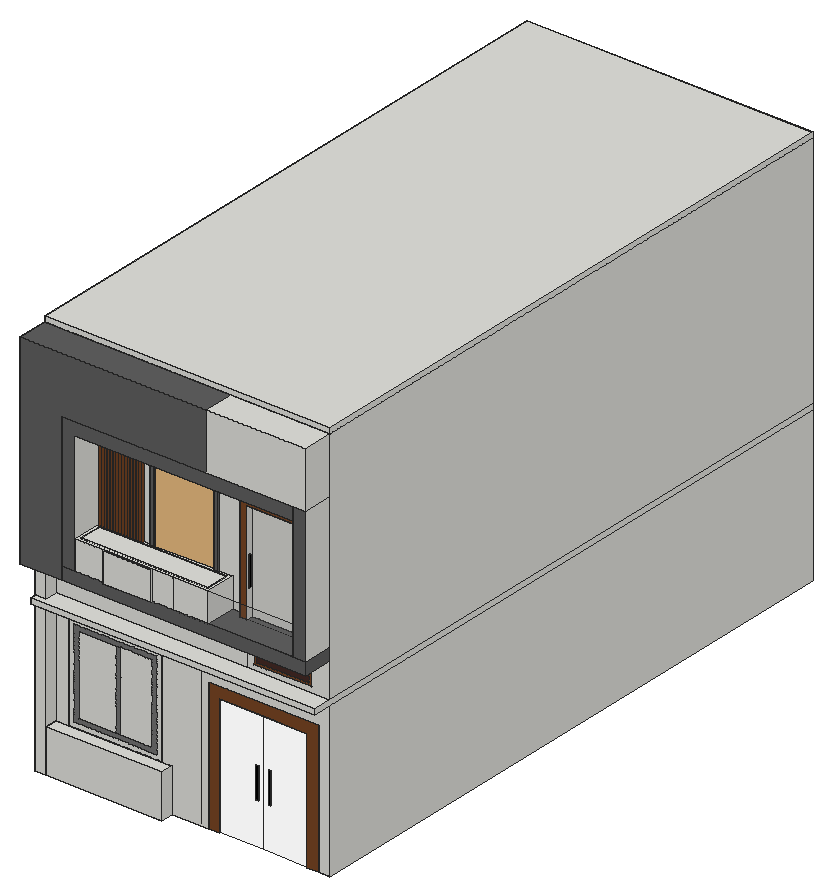
# SketchUp Ruby script. Lengths in inches.
U = 1.inch
M = Sketchup.active_model
def pt(a) = Geom::Point3d.new(a.map { |v| v * U })
def face(e, loops, mat)
  f = e.add_face(loops[0].map { |a| pt(a) })
  loops[1..].each { |l| e.add_face(l.map { |a| pt(a) }).erase! }
  f.material = f.back_material = mat if mat
  f
end
# faces: each face lists its corners as indices into pts; further lists are holes
def faces(e, pts, list, mat = nil) = list.each { |f| face(e, (f[0].is_a?(Array) ? f : [f]).map { |l| l.map { |i| pts[i] } }, mat) }
# xy, xz, yz: faces in a plane at the given z, y or x. An outline is a flat list of corners, or four numbers for a rectangle; further outlines are holes
def ring(l) = l.size == 4 ? [[l[0], l[1]], [l[2], l[1]], [l[2], l[3]], [l[0], l[3]]] : l.each_slice(2).to_a
def flat(e, list, mat, &to3) = list.each { |f| face(e, (f[0].is_a?(Array) ? f : [f]).map { |l| ring(l).map { |u, v| to3.(u, v) } }, mat) }
def xy(e, z, list, mat = nil) = flat(e, list, mat) { |x, y| [x, y, z] }
def xz(e, y, list, mat = nil) = flat(e, list, mat) { |x, z| [x, y, z] }
def yz(e, x, list, mat = nil) = flat(e, list, mat) { |y, z| [x, y, z] }
def lines(e, pts, list) = list.each { |a, b| e.add_line(pt(pts[a]), pt(pts[b])) }
# prism: a flat outline (further loops are holes) pulled along v
def prism(e, loops, v, mat = nil)
  f = face(e, loops, mat); d = Geom::Vector3d.new(v.map { |x| x * U })
  f.pushpull(f.normal.samedirection?(d) ? d.length : -d.length)
end
def box(e, o, s, mat = nil) = prism(e, [[o, [o[0] + s[0], o[1], o[2]], [o[0] + s[0], o[1] + s[1], o[2]], [o[0], o[1] + s[1], o[2]]]], [0, 0, s[2]], mat)
def at(x, y, z, deg = 0) = Geom::Transformation.translation(pt([x, y, z])) * Geom::Transformation.rotation(ORIGIN, Z_AXIS, deg.degrees)
def axes(o, x, y, z) = Geom::Transformation.new([*x, 0, *y, 0, *z, 0, *pt(o).to_a, 1])
def part(name) = M.definitions.add(name)
# library, detail: a bought-in or finely detailed component or shape, given as its bounding box
def library(name, o, s) = part(name).tap { |d| box(d.entities, o, s) }
def detail(e, o, s) = box(e.add_group.entities, o, s)
def put(e, d, t, mat = nil) = e.add_instance(d, t).tap { |i| i.material = mat if mat }
def group(e, t, mat = nil) = e.add_group.tap { |g| g.transformation = t; g.material = mat if mat }.entities
root = M.entities
M.materials.add("Lily_Dark").color = [68, 42, 38]
M.materials.add("Material12").color = [68, 110, 58]
M.materials.add("Material13").color = [48, 90, 38]
M.materials.add("Material14").color = [68, 110, 48]
M.materials.add("Material15").color = [48, 90, 48]
M.materials.add("Material16").color = [58, 110, 58]
M.materials.add("Material17").color = [58, 90, 38]
M.materials.add("Material18").color = [68, 100, 58]
M.materials.add("Material19").color = [48, 100, 38]
M.materials.add("Material~1").color = [96, 96, 96]
M.materials.add("[Color M05]").color = [114, 114, 114]
M.materials.add("[Color M09]").color = [0, 0, 0]
M.materials.add("[Color_000]").color = [255, 255, 255]
M.materials.add("[Color_009]").color = [0, 0, 0]
M.materials.add("[Groundcover_BarkChips]").color = [119, 116, 116]
M.materials.add("[Translucent Glass Gray]").color = [128, 128, 128]
M.materials["[Translucent Glass Gray]"].alpha = 0.1
M.materials.add("[Wood Veneer 01]").color = [120, 70, 37]
M.materials.add("stainless-steel").color = [0, 0, 0]
c1 = part("Corrugated panel")
box(c1.entities,[0,-2,0],[0.29,2,87.84])
box(c1.entities,[2.25,-2,0],[0.29,2,87.84])
box(c1.entities,[4.5,-2,0],[0.29,2,87.84])
box(c1.entities,[6.75,-2,0],[0.29,2,87.84])
box(c1.entities,[9,-2,0],[0.29,2,87.84])
box(c1.entities,[11.25,-2,0],[0.29,2,87.84])
box(c1.entities,[13.5,-2,0],[0.29,2,87.84])
box(c1.entities,[15.75,-2,0],[0.29,2,87.84])
box(c1.entities,[18,-2,0],[0.29,2,87.84])
box(c1.entities,[20.25,-2,0],[0.29,2,87.84])
box(c1.entities,[22.5,-2,0],[0.29,2,87.84])
box(c1.entities,[24.75,-2,0],[0.29,2,87.84])
box(c1.entities,[27,-2,0],[0.29,2,87.84])
box(c1.entities,[29.25,-2,0],[0.29,2,87.84])
box(c1.entities,[31.5,-2,0],[0.29,2,87.84])
box(c1.entities,[33.75,-2,0],[0.29,2,87.84])
box(c1.entities,[36,-2,0],[0.29,2,87.84])
box(c1.entities,[38.25,-2,0],[0.29,2,87.84])
box(c1.entities,[40.5,-2,0],[0.29,2,87.84])
box(c1.entities,[42.75,-2,0],[0.29,2,87.84])
box(c1.entities,[45,-2,0],[0.29,2,87.84])
c2 = library("Entrance door assembly",[-0.84,0,0],[9.1,39.62,78.08])
c3 = part("grass00")
p = [[-0.6875,0.15,0],[-0.56,0.08,5.52],[-0.04,0.03,2.76],[0.48,-0.02,0],[0.35,-0.02,5.52],[-0.1,-0.14,5.52],
  [-0.12,0.65,8.37],[-0.42,0.65,8.37]]
faces(c3.entities,p,[[0,1,2,3],[3,2,4],[1,5,2],[5,4,2],[1,6,5],[4,5,6],[7,6,1]])
c4 = part("Group108\#1")
put(c4.entities,c3,axes([-0.58,1.48,-0.01],[-0.26105,-0.10256,0],[0.0935,-0.23799,0.11527],[-0.04215,0.10729,0.25569]),"Material13")
put(c4.entities,c3,axes([-0.52,0.79,-0.01],[-0.30673,-0.20262,0],[0.17042,-0.25799,0.19884],[-0.1096,0.16591,0.30919]),"Material19")
put(c4.entities,c3,axes([-1.29,1.27,-0.01],[-0.1009,-0.10249,0],[0.10193,-0.10034,0.01514],[-0.01079,0.01062,0.14303]),"Material12")
put(c4.entities,c3,axes([-1.58,1.01,-0.01],[-0.09481,-0.14853,0],[0.12966,-0.08276,0.08597],[-0.07246,0.04626,0.15382]))
put(c4.entities,c3,axes([-0.85,0.32,-0.01],[-0.07211,-0.19233,0],[0.17265,-0.06473,0.09052],[-0.08476,0.03178,0.18439]),"Material16")
put(c4.entities,c3,axes([-1.06,0.16,-0.01],[-0.03023,-0.20103,0],[0.19643,-0.02954,0.04326],[-0.04278,0.00643,0.19863]),"Material17")
put(c4.entities,c3,axes([-1.78,-0.11,-0.01],[0.01133,-0.18805,0],[0.18159,0.01094,0.04894],[-0.04885,-0.00294,0.18192]),"Material19")
put(c4.entities,c3,axes([-1.57,-0.43,-0.01],[0.06705,-0.24264,0],[0.22711,0.06276,0.08862],[-0.08542,-0.02361,0.23562]),"Material14")
put(c4.entities,c3,axes([-0.97,-0.51,-0.01],[0.07163,-0.1379,0],[0.1379,0.07163,0.00033],[-0.00029,-0.00015,0.15539]),"Material16")
put(c4.entities,c3,axes([-0.55,-0.45,-0.01],[0.22039,-0.26784,0],[0.17095,0.14066,0.26702],[-0.20619,-0.16966,0.22138]),"Material19")
put(c4.entities,c3,axes([-0.66,-0.83,-0.01],[0.15006,-0.11959,0],[0.10592,0.13291,0.08908],[-0.05552,-0.06966,0.16995]),"Material19")
put(c4.entities,c3,axes([-0.36,-0.72,-0.01],[0.33439,-0.1671,0],[0.1176,0.23533,0.26558],[-0.11871,-0.23757,0.26308]),"Material12")
put(c4.entities,c3,axes([-0.17,-0.64,-0.01],[0.32333,-0.08393,0],[0.04214,0.16232,0.2889],[-0.07259,-0.27963,0.1677]))
put(c4.entities,c3,axes([-0.04,-0.9,-0.01],[0.26603,-0.01186,0],[0.01186,0.26603,0.00131],[-0.00006,-0.00131,0.26629]),"Material16")
put(c4.entities,c3,axes([0.21,-1.24,-0.01],[0.19373,0.03224,0],[-0.02742,0.16477,0.10329],[0.01696,-0.10189,0.16703]))
put(c4.entities,c3,axes([0.58,-1.47,-0.01],[0.27421,0.10773,0],[-0.06718,0.171,0.23031],[0.08421,-0.21436,0.18372]),"Material17")
put(c4.entities,c3,axes([1.01,-1.53,-0.01],[0.182,0.12023,0],[-0.11708,0.17724,0.04956],[0.02732,-0.04135,0.21242]),"Material15")
put(c4.entities,c3,axes([1.13,-1.11,-0.01],[0.08993,0.09135,0],[-0.04886,0.0481,0.10832],[0.07719,-0.07599,0.06856]),"Material16")
put(c4.entities,c3,axes([0.57,-0.37,-0.01],[0.13107,0.20532,0],[-0.17134,0.10937,0.13423],[0.11314,-0.07222,0.20327]),"Material14")
put(c4.entities,c3,axes([1.17,-0.44,-0.01],[0.12226,0.32609,0],[-0.18227,0.06833,0.28877],[0.27039,-0.10137,0.19466]),"Material12")
put(c4.entities,c3,axes([0.79,-0.12,-0.01],[0.04726,0.31426,0],[-0.23697,0.03563,0.20873],[0.20641,-0.03104,0.23963]),"Material13")
put(c4.entities,c3,axes([1.11,0.07,-0.01],[-0.00983,0.16317,0],[-0.12959,-0.00781,0.09932],[0.09914,0.00597,0.12983]),"Material15")
put(c4.entities,c3,axes([1.34,0.37,-0.01],[-0.077,0.27862,0],[-0.26284,-0.07264,0.09592],[0.09245,0.02555,0.27269]),"Material18")
put(c4.entities,c3,axes([1.43,0.74,-0.01],[-0.09818,0.18902,0],[-0.17019,-0.0884,0.09267],[0.08224,0.04272,0.19178]),"Material15")
put(c4.entities,c3,axes([0.68,0.56,-0.01],[-0.19396,0.23573,0],[-0.19529,-0.16069,0.17096],[0.13201,0.10862,0.2529]),"Material17")
put(c4.entities,c3,axes([1.13,1.42,-0.01],[-0.175,0.13946,0],[-0.12896,-0.16183,0.08516],[0.05308,0.0666,0.20693]),"Material19")
put(c4.entities,c3,axes([0.57,1.15,-0.01],[-0.14357,0.07174,0],[-0.03981,-0.07966,0.13353],[0.05969,0.11944,0.08905]),"Material19")
put(c4.entities,c3,axes([0.42,1.63,-0.01],[-0.19191,0.04982,0],[-0.03576,-0.13775,0.13805],[0.03469,0.13362,0.14232]))
put(c4.entities,c3,axes([0.05,1.02,-0.01],[-0.23102,0.0103,0],[-0.00712,-0.15969,0.1671],[0.00744,0.16694,0.15985]),"Material12")
put(c4.entities,c3,axes([-0.24,1.45,-0.01],[-0.18944,-0.03152,0],[0.03127,-0.1879,0.02439],[-0.004,0.02405,0.19049]),"Material15")
c5 = part("Group107\#1")
put(c5.entities,c4,at(0,0,0))
c6 = part("3darcstudiotree_grass00")
put(c6.entities,c5,at(0,0,0))
c7 = part("Group104\#1")
put(c7.entities,c6,axes([121.2,-0.39,1.37],[-1.04345,0.21132,0],[-0.2343,-1.15691,-0.03532],[-0.00931,-0.04597,1.5674]))
put(c7.entities,c6,axes([126.74,-0.5,1.37],[-0.81222,-0.535,0],[0.66881,-1.01537,-0.05333],[0.03791,-0.05756,1.57138]))
put(c7.entities,c6,axes([116.24,-0.29,1.37],[0.45586,-0.8369,0],[1.087,0.59209,-0.05145],[0.05418,0.02951,1.48449]))
put(c7.entities,c6,axes([129.92,-1.13,1.37],[0.5987,0.96121,0],[-0.80897,0.50387,-0.01309],[-0.01852,0.01154,1.58919]))
put(c7.entities,c6,axes([112.39,-0.41,1.37],[-0.41741,-1.14553,0],[0.92662,-0.33764,-0.04573],[0.06587,-0.024,1.51206]))
put(c7.entities,c6,axes([132.01,-1.1,1.37],[1.1241,-0.29373,0],[0.24406,0.934,-0.01529],[0.00612,0.02342,1.52853]))
put(c7.entities,c6,axes([109.24,-1.23,1.37],[0.10575,1.00852,0],[-1.03726,0.10876,-0.00707],[-0.01059,0.00111,1.57151]))
put(c7.entities,c6,axes([123.48,-1.1875,1.37],[-1.04345,0.21132,0],[-0.2343,-1.15691,-0.03532],[-0.00931,-0.04597,1.5674]))
put(c7.entities,c6,axes([119.28,-1.1875,1.37],[-1.04345,0.21132,0],[-0.2343,-1.15691,-0.03532],[-0.00931,-0.04597,1.5674]))
put(c7.entities,c6,axes([115.03,-1.13,1.37],[0.45586,-0.8369,0],[1.087,0.59209,-0.05145],[0.05418,0.02951,1.48449]))
c8 = part("Grass planter")
xy(c8.entities,0,[[[0.37,1.03,27.93,6.94],[0.77,1.43,27.54,6.55]]],"[Color_000]")
xy(c8.entities,1.37,[[0.77,1.43,27.54,6.55]],"[Groundcover_BarkChips]")
xy(c8.entities,1.57,[[[0.37,1.03,27.93,6.94],[0.77,1.43,27.54,6.55]]],"[Color_009]")
xz(c8.entities,1.03,[[0.37,0,27.93,1.57]])
xz(c8.entities,1.43,[[0.77,0,27.54,1.37]],"[Color_000]")
xz(c8.entities,1.43,[[0.77,1.37,27.54,1.57]],"[Color_009]")
xz(c8.entities,6.55,[[0.77,0,27.54,1.37]],"[Color_000]")
xz(c8.entities,6.55,[[0.77,1.37,27.54,1.57]],"[Color_009]")
xz(c8.entities,6.94,[[0.37,0,27.93,1.57]])
yz(c8.entities,0.37,[[1.03,0,6.94,1.57]])
yz(c8.entities,0.77,[[1.43,0,6.55,1.37]],"[Color_000]")
yz(c8.entities,0.77,[[1.43,1.37,6.55,1.57]],"[Color_009]")
yz(c8.entities,27.54,[[1.43,0,6.55,1.37]],"[Color_000]")
yz(c8.entities,27.54,[[1.43,1.37,6.55,1.57]],"[Color_009]")
yz(c8.entities,27.93,[[1.03,0,6.94,1.57]])
put(c8.entities,c7,at(-106.55,4.625,0))
c9 = part("Difference\#2")
xy(c9.entities,0,[[0,0,0,473,223.84,473,223.84,0,214.84,0,214.84,464,9,464,9,9,128.52,9,128.52,0]])
xy(c9.entities,34,[[19.21,0,92.04,9]])
xy(c9.entities,103,[[128.52,0,214.84,9]])
xy(c9.entities,111,[[19.21,0,92.04,9]])
xy(c9.entities,120,[[[0,0,223.84,473],[9,9,214.84,464]]])
xz(c9.entities,0,[[[0,0,128.52,0,128.52,103,214.84,103,214.84,0,223.84,0,223.84,120,0,120],[19.21,34,92.04,111]]])
xz(c9.entities,9,[[[9,0,9,120,214.84,120,214.84,103,128.52,103,128.52,0],[19.21,34,92.04,111]]])
xz(c9.entities,464,[[9,0,214.84,120]])
xz(c9.entities,473,[[0,0,223.84,120]])
yz(c9.entities,0,[[0,0,473,120]])
yz(c9.entities,9,[[9,0,464,120]])
yz(c9.entities,19.21,[[0,34,9,111]])
yz(c9.entities,92.04,[[0,34,9,111]])
yz(c9.entities,128.52,[[0,0,9,103]])
yz(c9.entities,214.84,[[0,0,9,103],[9,0,464,120]])
yz(c9.entities,223.84,[[0,0,473,120]])
p = [[123.02,0,1.98],[123.02,0,120]]
lines(c9.entities,p,[[0,1]])
c10 = part("Difference\#1")
xy(c10.entities,0,[[0,0,0,473,223.84,473,223.84,0,128.52,0,128.52,9,214.84,9,214.84,464,9,464,9,9,128.52,9,128.52,0]])
xy(c10.entities,48.19,[[86.57,0,133.57,9]])
xy(c10.entities,122.19,[[86.57,0,133.57,9]])
xy(c10.entities,187,[[[0,0,223.84,473],[9,9,214.84,464]]])
xz(c10.entities,0,[[[0,0,158.62,0,158.62,27.47,223.84,27.47,223.84,187,0,187],[86.57,48.19,133.57,122.19]]])
xz(c10.entities,9,[[[9,0,214.84,187],[86.57,48.19,133.57,122.19]]])
xz(c10.entities,464,[[9,0,214.84,187]])
xz(c10.entities,473,[[0,0,223.84,187]])
yz(c10.entities,0,[[0,0,473,187]])
yz(c10.entities,9,[[9,0,464,187]])
yz(c10.entities,86.57,[[0,48.19,9,122.19]])
yz(c10.entities,133.57,[[0,48.19,9,122.19]])
yz(c10.entities,214.84,[[9,0,464,187]])
yz(c10.entities,223.84,[[0,0,473,187]])
p = [[124.34,0,27.47],[119.51,0,27.47],[131.53,0,27.47],[126.28,0,27.47]]
lines(c10.entities,p,[[0,1],[2,3]])
g1 = group(c10.entities,at(158.62,0,0))
xz(g1,0,[[[0,0,65.22,27.47],[5.85,3.79,50.85,21.79]]])
xz(g1,0,[[8.1,6.04,48.6,19.54]],"Lily_Dark")
xz(g1,0,[[[5.85,3.79,50.85,21.79],[8.1,6.04,48.6,19.54]]],"[Wood Veneer 01]")
prism(root,[[[86.44,25,171.48],[86.44,25,168.05],[83.01,25,168.05],[83.01,25,251.05],[137.01,25,251.05],[137.01,25,168.05],[133.57,25,168.05],[133.57,25,246.19],[86.44,25,246.19]]],[0,-1,0],"Material~1")
box(root,[0,25,311],[223.84,473,4])
xy(root,161.23,[[32.8,1,42.57,25],[214.07,1,223.84,25]])
xy(root,256.55,[[42.57,1,214.07,25]])
xy(root,266.3125,[[32.8,1,214.07,25],[214.07,1,223.84,25]])
xz(root,1,[[32.8,161.23,42.57,161.23,42.57,256.55,214.07,256.55,214.07,266.3125,32.8,266.3125],[214.07,161.23,223.84,266.3125]],"Material~1")
xz(root,1,[[147.49,161.23,214.07,184.23]],"[Translucent Glass Gray]")
xz(root,20,[[162.77,161.23,198.8,241.27]],"[Translucent Glass Gray]")
xz(root,25,[[[19.21,34,92.04,111],[23.14,37.92,88.12,107.08]],[26.85,41.63,55.625,103.37],[60.03,41.63,84.41,103.37],[32.8,161.23,32.8,266.3125,214.07,266.3125,214.07,256.55,42.57,256.55,42.57,161.23],[214.07,161.23,223.84,266.3125]])
xz(root,25,[[[23.14,37.92,88.12,107.08],[26.85,41.63,84.41,103.37]],[55.625,41.63,60.03,103.37]],"[Color M05]")
xz(root,25,[[165.65,33.6,167.65,57.6],[175.65,33.6,177.65,57.6]],"[Color M09]")
xz(root,25,[[[137.43,0,171.68,94.08],[165.65,33.6,167.65,57.6]],[[171.68,0,205.92,94.08],[175.65,33.6,177.65,57.6]]],"[Translucent Glass Gray]")
xz(root,25,[[128.52,0,137.43,0,137.43,94.08,205.92,94.08,205.92,0,214.84,0,214.84,103,128.52,103]],"[Wood Veneer 01]")
yz(root,32.8,[[1,161.23,25,266.3125]])
yz(root,42.57,[[1,161.23,25,256.55]])
yz(root,214.07,[[1,161.23,25,256.55],[1,256.55,25,266.3125]])
yz(root,223.84,[[1,161.23,25,266.3125]])
put(root,c1,at(32.8,25,171.47),"[Wood Veneer 01]")
put(root,c2,axes([87.05,29.48,172.19],[0.02104,-0.63409,0],[1.16936,0.03879,0],[0,0,0.94779]))
put(root,c8,at(0,25,0))
put(root,c9,at(0,25,0))
g2 = group(root,at(0,25,120))
prism(g2,[[[0,0,0],[0,473,0],[223.84,473,0],[223.84,-15,0],[1,-15,0],[1,0,0]]],[0,0,4])
put(root,c10,at(0,25,124))
g3 = group(root,at(0,25,-20))
g4 = group(g3,at(0,-2,0))
box(g4,[0,-8,20],[9,10,151.47])
g5 = group(root,at(0,25,171.47))
xy(g5,-20,[[0,-24,32.8,0]])
xy(g5,94.84,[[32.8,-24,223.84,0]])
xy(g5,139.53,[[146.04,-24,223.84,0]])
xy(g5,139.53,[[0,-24,146.04,0]],"Material~1")
xz(g5,-24,[[146.04,94.84,223.84,139.53]])
xz(g5,-24,[[0,-20,32.8,-20,32.8,94.84,146.04,94.84,146.04,139.53,0,139.53]],"Material~1")
xz(g5,0,[[0,-20,0,139.53,223.84,139.53,223.84,94.84,32.8,94.84,32.8,-20]])
yz(g5,0,[[-24,-20,0,139.53]],"Material~1")
yz(g5,32.8,[[-24,-20,0,94.84]])
yz(g5,223.84,[[-24,94.84,0,139.53]])
g6 = group(root,at(32.8,1,151.47),"Material~1")
prism(g6,[[[181.27,0,9.76],[9.76,0,9.76],[0,0,9.76],[0,0,0],[191.03,0,0],[191.03,0,9.76]]],[0,24,0])
g7 = group(root,at(42.57,1,161.23))
xy(g7,0,[[23.43,-1,60.69,0],[0,0,104.93,24]])
xy(g7,23,[[23.43,-1,60.69,0],[[0,0,104.93,24],[2.68,2.68,102.25,21.32]],[2.68,2.68,102.25,21.32]])
xz(g7,-1,[[23.43,0,60.69,23]])
xz(g7,0,[[0,0,23.43,23],[23.43,0,60.69,23],[60.69,0,76.98,23],[76.98,0,104.93,23]])
xz(g7,2.68,[[2.68,18,23.43,23],[23.43,18,60.69,23],[60.69,18,76.98,23],[76.98,18,102.25,23]])
xz(g7,21.32,[[2.68,18,102.25,23]])
yz(g7,0,[[0,0,24,23]])
yz(g7,2.68,[[2.68,18,21.32,23]])
yz(g7,23.43,[[-1,0,0,23]])
yz(g7,60.69,[[-1,0,0,23]])
yz(g7,102.25,[[2.68,18,21.32,23]])
yz(g7,104.93,[[0,0,24,23]])
g8 = group(root,at(147.49,25,161.23))
xy(g8,0,[[9.38,-5,15.28,0],[51.31,-5,57.2,0],[15.28,0,51.31,9]])
xy(g8,80.04,[[15.28,-5,51.31,9]])
xy(g8,85.93,[[9.38,-5,57.2,0]])
xz(g8,-5,[[9.38,0,15.28,0,15.28,80.04,51.31,80.04,51.31,0,57.2,0,57.2,85.93,9.38,85.93]],"[Wood Veneer 01]")
xz(g8,0,[[0,0,9.38,0,9.38,85.93,57.2,85.93,57.2,0,66.58,0,66.58,95.32,0,95.32]])
xz(g8,9,[[15.28,0,51.31,80.04]])
yz(g8,9.38,[[-5,0,0,85.93]])
yz(g8,15.28,[[-5,0,9,80.04]])
yz(g8,51.31,[[-5,0,9,80.04]])
yz(g8,57.2,[[-5,0,0,85.93]])
g9 = group(root,at(165.05,20,184.9))
box(g9,[0,-1,0],[1,1,23],"stainless-steel")
g10 = group(root,at(9,25,0))
box(g10,[0,-10,0],[91,10,34])
